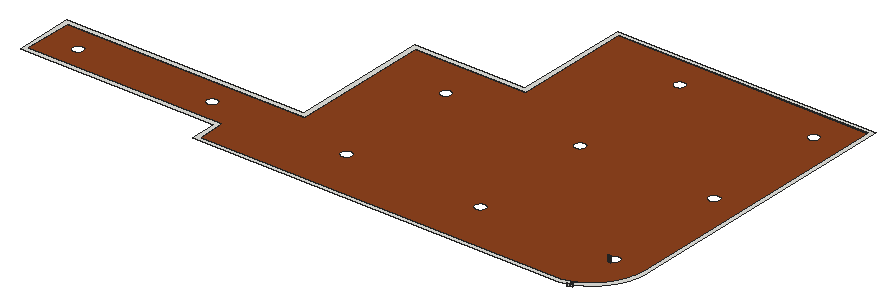
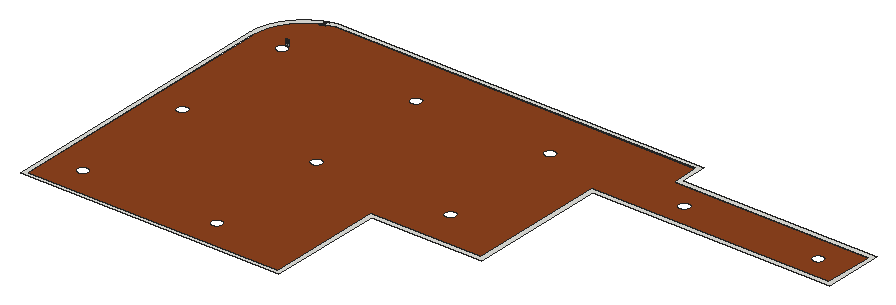
# SketchUp Ruby script. Lengths in inches.
U = 1.inch
M = Sketchup.active_model
def pt(a) = Geom::Point3d.new(a.map { |v| v * U })
def face(e, loops, mat)
  f = e.add_face(loops[0].map { |a| pt(a) })
  loops[1..].each { |l| e.add_face(l.map { |a| pt(a) }).erase! }
  f.material = f.back_material = mat if mat
  f
end
# faces: each face lists its corners as indices into pts; further lists are holes
def faces(e, pts, list, mat = nil) = list.each { |f| face(e, (f[0].is_a?(Array) ? f : [f]).map { |l| l.map { |i| pts[i] } }, mat) }
# xy, xz, yz: faces in a plane at the given z, y or x. An outline is a flat list of corners, or four numbers for a rectangle; further outlines are holes
def ring(l) = l.size == 4 ? [[l[0], l[1]], [l[2], l[1]], [l[2], l[3]], [l[0], l[3]]] : l.each_slice(2).to_a
def flat(e, list, mat, &to3) = list.each { |f| face(e, (f[0].is_a?(Array) ? f : [f]).map { |l| ring(l).map { |u, v| to3.(u, v) } }, mat) }
def xy(e, z, list, mat = nil) = flat(e, list, mat) { |x, y| [x, y, z] }
def xz(e, y, list, mat = nil) = flat(e, list, mat) { |x, z| [x, y, z] }
def yz(e, x, list, mat = nil) = flat(e, list, mat) { |y, z| [x, y, z] }
def lines(e, pts, list) = list.each { |a, b| e.add_line(pt(pts[a]), pt(pts[b])) }
# prism: a flat outline (further loops are holes) pulled along v
def prism(e, loops, v, mat = nil)
  f = face(e, loops, mat); d = Geom::Vector3d.new(v.map { |x| x * U })
  f.pushpull(f.normal.samedirection?(d) ? d.length : -d.length)
end
def box(e, o, s, mat = nil) = prism(e, [[o, [o[0] + s[0], o[1], o[2]], [o[0] + s[0], o[1] + s[1], o[2]], [o[0], o[1] + s[1], o[2]]]], [0, 0, s[2]], mat)
def at(x, y, z, deg = 0) = Geom::Transformation.translation(pt([x, y, z])) * Geom::Transformation.rotation(ORIGIN, Z_AXIS, deg.degrees)
def axes(o, x, y, z) = Geom::Transformation.new([*x, 0, *y, 0, *z, 0, *pt(o).to_a, 1])
def part(name) = M.definitions.add(name)
# library, detail: a bought-in or finely detailed component or shape, given as its bounding box
def library(name, o, s) = part(name).tap { |d| box(d.entities, o, s) }
def detail(e, o, s) = box(e.add_group.entities, o, s)
def put(e, d, t, mat = nil) = e.add_instance(d, t).tap { |i| i.material = mat if mat }
def group(e, t, mat = nil) = e.add_group.tap { |g| g.transformation = t; g.material = mat if mat }.entities
root = M.entities
M.materials.add("[Wood Fence]").color = [142, 67, 30]
xy(root,108,[[[135.5,161,135.5,175,35,175,35,201,158,201,158,273,215,273,215,333,345,333,345,186.92,344.99,186.68,344.98,186.4375,344.97,186.2,344.95,185.72,344.93,185.48,344.91,185.25,344.87,184.77,344.84,184.53,344.8125,184.29,344.78,184.06,344.72,183.58,344.68,183.35,344.64,183.11,344.6,182.875,344.5625,182.64,344.52,182.4,344.47,182.17,344.42,181.93,344.375,181.7,344.32,181.47,344.27,181.23,344.03,180.31,343.96,180.08,343.9,179.85,343.76,179.39,343.68,179.16,343.61,178.9375,343.53,178.71,343.45,178.48,343.375,178.26,343.29,178.03,343.21,177.81,343.03,177.37,342.94,177.14,342.85,176.92,342.75,176.7,342.66,176.48,342.56,176.27,342.46,176.05,342.35,175.83,342.25,175.62,342.14,175.4,342.04,175.19,341.93,174.98,341.8125,174.77,341.7,174.56,341.58,174.35,341.47,174.14,341.23,173.72,341.1,173.52,340.98,173.32,340.85,173.11,340.46,172.51,340.33,172.3125,340.19,172.12,340.06,171.92,339.92,171.72,339.78,171.53,339.63,171.34,339.49,171.15,339.34,170.96,339.2,170.77,339.05,170.58,338.9,170.4,338.75,170.21,338.59,170.03,338.4375,169.85,338.28,169.67,338.12,169.49,337.96,169.3125,337.8,169.13,337.63,168.96,337.47,168.79,337.3,168.62,337.13,168.44,336.97,168.28,336.79,168.11,336.62,167.94,336.45,167.78,336.27,167.62,336.1,167.46,335.56,166.98,335.375,166.83,335.19,166.67,335.01,166.52,334.63,166.22,334.44,166.08,334.25,165.93,333.87,165.65,333.67,165.51,333.48,165.37,333.28,165.23,332.08,164.45,331.87,164.33,331.67,164.21,331.04,163.85,330.83,163.74,330.62,163.625,330.41,163.52,330.2,163.41,329.98,163.3,329.77,163.19,329.55,163.09,329.34,162.99,328.9,162.79,328.68,162.7,328.46,162.6,328.02,162.42,327.79,162.34,327.57,162.25,327.35,162.17,327.12,162.08,326.9,162,326.67,161.93,326.44,161.85,326.22,161.78,325.99,161.7,325.76,161.64,325.3,161.5,324.84,161.375,324.61,161.32,324.14,161.2,323.68,161.1,323.44,161.05,323.21,161],[120.34,185,120.66,185,120.74,185.01,120.8125,185.02,120.89,185.03,121.05,185.05,121.125,185.07,121.2,185.08,121.28,185.1,121.35,185.125,121.43,185.15,121.5,185.17,121.58,185.2,121.79,185.29,121.86,185.33,121.93,185.36,122.07,185.44,122.13,185.48,122.2,185.53,122.26,185.57,122.33,185.62,122.57,185.82,122.62,185.88,122.68,185.93,122.88,186.17,122.93,186.24,122.97,186.3,123.02,186.37,123.06,186.43,123.14,186.57,123.17,186.64,123.21,186.71,123.3,186.92,123.33,187,123.35,187.07,123.375,187.15,123.4,187.22,123.42,187.3,123.43,187.375,123.45,187.45,123.47,187.61,123.48,187.6875,123.49,187.76,123.5,187.84,123.5,188.16,123.49,188.24,123.48,188.3125,123.47,188.39,123.45,188.55,123.43,188.625,123.42,188.7,123.4,188.78,123.375,188.85,123.35,188.93,123.33,189,123.3,189.08,123.21,189.29,123.17,189.36,123.14,189.43,123.06,189.57,123.02,189.63,122.97,189.7,122.93,189.76,122.88,189.83,122.68,190.07,122.62,190.12,122.57,190.18,122.33,190.38,122.26,190.43,122.2,190.47,122.13,190.52,122.07,190.56,121.93,190.64,121.86,190.67,121.79,190.71,121.58,190.8,121.5,190.83,121.43,190.85,121.35,190.875,121.28,190.9,121.2,190.92,121.125,190.93,121.05,190.95,120.89,190.97,120.8125,190.98,120.74,190.99,120.66,191,120.34,191,120.26,190.99,120.1875,190.98,120.11,190.97,119.95,190.95,119.875,190.93,119.8,190.92,119.72,190.9,119.65,190.875,119.57,190.85,119.5,190.83,119.42,190.8,119.21,190.71,119.14,190.67,119.07,190.64,118.93,190.56,118.87,190.52,118.8,190.47,118.74,190.43,118.67,190.38,118.43,190.18,118.38,190.12,118.32,190.07,118.12,189.83,118.07,189.76,118.03,189.7,117.98,189.63,117.94,189.57,117.86,189.43,117.83,189.36,117.79,189.29,117.7,189.08,117.67,189,117.65,188.93,117.625,188.85,117.6,188.78,117.58,188.7,117.57,188.625,117.55,188.55,117.53,188.39,117.52,188.3125,117.51,188.24,117.5,188.16,117.5,187.84,117.51,187.76,117.52,187.6875,117.53,187.61,117.55,187.45,117.57,187.375,117.58,187.3,117.6,187.22,117.625,187.15,117.65,187.07,117.67,187,117.7,186.92,117.79,186.71,117.83,186.64,117.86,186.57,117.94,186.43,117.98,186.37,118.03,186.3,118.07,186.24,118.12,186.17,118.32,185.93,118.38,185.88,118.43,185.82,118.67,185.62,118.74,185.57,118.8,185.53,118.87,185.48,118.93,185.44,119.07,185.36,119.14,185.33,119.21,185.29,119.42,185.2,119.5,185.17,119.57,185.15,119.65,185.125,119.72,185.1,119.8,185.08,119.875,185.07,119.95,185.05,120.11,185.03,120.1875,185.02,120.26,185.01],[259.34,314,259.66,314,259.74,314.01,259.8125,314.02,259.89,314.03,260.05,314.05,260.125,314.07,260.2,314.08,260.28,314.1,260.35,314.125,260.43,314.15,260.5,314.17,260.58,314.2,260.79,314.29,260.86,314.33,260.93,314.36,261.07,314.44,261.13,314.48,261.2,314.53,261.26,314.57,261.33,314.62,261.57,314.82,261.62,314.88,261.68,314.93,261.88,315.17,261.93,315.24,261.97,315.3,262.02,315.37,262.06,315.43,262.14,315.57,262.17,315.64,262.21,315.71,262.3,315.92,262.33,316,262.35,316.07,262.375,316.15,262.4,316.22,262.42,316.3,262.43,316.375,262.45,316.45,262.47,316.61,262.48,316.6875,262.49,316.76,262.5,316.84,262.5,317.16,262.49,317.24,262.48,317.3125,262.47,317.39,262.45,317.55,262.43,317.625,262.42,317.7,262.4,317.78,262.375,317.85,262.35,317.93,262.33,318,262.3,318.08,262.21,318.29,262.17,318.36,262.14,318.43,262.06,318.57,262.02,318.63,261.97,318.7,261.93,318.76,261.88,318.83,261.68,319.07,261.62,319.12,261.57,319.18,261.33,319.38,261.26,319.43,261.2,319.47,261.13,319.52,261.07,319.56,260.93,319.64,260.86,319.67,260.79,319.71,260.58,319.8,260.5,319.83,260.43,319.85,260.35,319.875,260.28,319.9,260.2,319.92,260.125,319.93,260.05,319.95,259.89,319.97,259.8125,319.98,259.74,319.99,259.66,320,259.34,320,259.26,319.99,259.1875,319.98,259.11,319.97,258.95,319.95,258.875,319.93,258.8,319.92,258.72,319.9,258.65,319.875,258.57,319.85,258.5,319.83,258.42,319.8,258.21,319.71,258.14,319.67,258.07,319.64,257.93,319.56,257.87,319.52,257.8,319.47,257.74,319.43,257.67,319.38,257.43,319.18,257.38,319.12,257.32,319.07,257.12,318.83,257.07,318.76,257.03,318.7,256.98,318.63,256.94,318.57,256.86,318.43,256.83,318.36,256.79,318.29,256.7,318.08,256.67,318,256.65,317.93,256.625,317.85,256.6,317.78,256.58,317.7,256.57,317.625,256.55,317.55,256.53,317.39,256.52,317.3125,256.51,317.24,256.5,317.16,256.5,316.84,256.51,316.76,256.52,316.6875,256.53,316.61,256.55,316.45,256.57,316.375,256.58,316.3,256.6,316.22,256.625,316.15,256.65,316.07,256.67,316,256.7,315.92,256.79,315.71,256.83,315.64,256.86,315.57,256.94,315.43,256.98,315.37,257.03,315.3,257.07,315.24,257.12,315.17,257.32,314.93,257.38,314.88,257.43,314.82,257.67,314.62,257.74,314.57,257.8,314.53,257.87,314.48,257.93,314.44,258.07,314.36,258.14,314.33,258.21,314.29,258.42,314.2,258.5,314.17,258.57,314.15,258.65,314.125,258.72,314.1,258.8,314.08,258.875,314.07,258.95,314.05,259.11,314.03,259.1875,314.02,259.26,314.01],[328.84,314,329.16,314,329.24,314.01,329.3125,314.02,329.39,314.03,329.55,314.05,329.625,314.07,329.7,314.08,329.78,314.1,329.85,314.125,329.93,314.15,330,314.17,330.08,314.2,330.29,314.29,330.36,314.33,330.43,314.36,330.57,314.44,330.63,314.48,330.7,314.53,330.76,314.57,330.83,314.62,331.07,314.82,331.12,314.88,331.18,314.93,331.38,315.17,331.43,315.24,331.47,315.3,331.52,315.37,331.56,315.43,331.64,315.57,331.67,315.64,331.71,315.71,331.8,315.92,331.83,316,331.85,316.07,331.875,316.15,331.9,316.22,331.92,316.3,331.93,316.375,331.95,316.45,331.97,316.61,331.98,316.6875,331.99,316.76,332,316.84,332,317.16,331.99,317.24,331.98,317.3125,331.97,317.39,331.95,317.55,331.93,317.625,331.92,317.7,331.9,317.78,331.875,317.85,331.85,317.93,331.83,318,331.8,318.08,331.71,318.29,331.67,318.36,331.64,318.43,331.56,318.57,331.52,318.63,331.47,318.7,331.43,318.76,331.38,318.83,331.18,319.07,331.12,319.12,331.07,319.18,330.83,319.38,330.76,319.43,330.7,319.47,330.63,319.52,330.57,319.56,330.43,319.64,330.36,319.67,330.29,319.71,330.08,319.8,330,319.83,329.93,319.85,329.85,319.875,329.78,319.9,329.7,319.92,329.625,319.93,329.55,319.95,329.39,319.97,329.3125,319.98,329.24,319.99,329.16,320,328.84,320,328.76,319.99,328.6875,319.98,328.61,319.97,328.45,319.95,328.375,319.93,328.3,319.92,328.22,319.9,328.15,319.875,328.07,319.85,328,319.83,327.92,319.8,327.71,319.71,327.64,319.67,327.57,319.64,327.43,319.56,327.37,319.52,327.3,319.47,327.24,319.43,327.17,319.38,326.93,319.18,326.88,319.12,326.82,319.07,326.62,318.83,326.57,318.76,326.53,318.7,326.48,318.63,326.44,318.57,326.36,318.43,326.33,318.36,326.29,318.29,326.2,318.08,326.17,318,326.15,317.93,326.125,317.85,326.1,317.78,326.08,317.7,326.07,317.625,326.05,317.55,326.03,317.39,326.02,317.3125,326.01,317.24,326,317.16,326,316.84,326.01,316.76,326.02,316.6875,326.03,316.61,326.05,316.45,326.07,316.375,326.08,316.3,326.1,316.22,326.125,316.15,326.15,316.07,326.17,316,326.2,315.92,326.29,315.71,326.33,315.64,326.36,315.57,326.44,315.43,326.48,315.37,326.53,315.3,326.57,315.24,326.62,315.17,326.82,314.93,326.88,314.88,326.93,314.82,327.17,314.62,327.24,314.57,327.3,314.53,327.37,314.48,327.43,314.44,327.57,314.36,327.64,314.33,327.71,314.29,327.92,314.2,328,314.17,328.07,314.15,328.15,314.125,328.22,314.1,328.3,314.08,328.375,314.07,328.45,314.05,328.61,314.03,328.6875,314.02,328.76,314.01],[259.34,249.5,259.66,249.5,259.74,249.51,259.8125,249.52,259.89,249.53,260.05,249.55,260.125,249.57,260.2,249.58,260.28,249.6,260.35,249.625,260.43,249.65,260.5,249.67,260.58,249.7,260.79,249.79,260.86,249.83,260.93,249.86,261.07,249.94,261.13,249.98,261.2,250.03,261.26,250.07,261.33,250.12,261.57,250.32,261.62,250.38,261.68,250.43,261.88,250.67,261.93,250.74,261.97,250.8,262.02,250.87,262.06,250.93,262.14,251.07,262.17,251.14,262.21,251.21,262.3,251.42,262.33,251.5,262.35,251.57,262.375,251.65,262.4,251.72,262.42,251.8,262.43,251.875,262.45,251.95,262.47,252.11,262.48,252.1875,262.49,252.26,262.5,252.34,262.5,252.66,262.49,252.74,262.48,252.8125,262.47,252.89,262.45,253.05,262.43,253.125,262.42,253.2,262.4,253.28,262.375,253.35,262.35,253.43,262.33,253.5,262.3,253.58,262.21,253.79,262.17,253.86,262.14,253.93,262.06,254.07,262.02,254.13,261.97,254.2,261.93,254.26,261.88,254.33,261.68,254.57,261.62,254.62,261.57,254.68,261.33,254.88,261.26,254.93,261.2,254.97,261.13,255.02,261.07,255.06,260.93,255.14,260.86,255.17,260.79,255.21,260.58,255.3,260.5,255.33,260.43,255.35,260.35,255.375,260.28,255.4,260.2,255.42,260.125,255.43,260.05,255.45,259.89,255.47,259.8125,255.48,259.74,255.49,259.66,255.5,259.34,255.5,259.26,255.49,259.1875,255.48,259.11,255.47,258.95,255.45,258.875,255.43,258.8,255.42,258.72,255.4,258.65,255.375,258.57,255.35,258.5,255.33,258.42,255.3,258.21,255.21,258.14,255.17,258.07,255.14,257.93,255.06,257.87,255.02,257.8,254.97,257.74,254.93,257.67,254.88,257.43,254.68,257.38,254.62,257.32,254.57,257.12,254.33,257.07,254.26,257.03,254.2,256.98,254.13,256.94,254.07,256.86,253.93,256.83,253.86,256.79,253.79,256.7,253.58,256.67,253.5,256.65,253.43,256.625,253.35,256.6,253.28,256.58,253.2,256.57,253.125,256.55,253.05,256.53,252.89,256.52,252.8125,256.51,252.74,256.5,252.66,256.5,252.34,256.51,252.26,256.52,252.1875,256.53,252.11,256.55,251.95,256.57,251.875,256.58,251.8,256.6,251.72,256.625,251.65,256.65,251.57,256.67,251.5,256.7,251.42,256.79,251.21,256.83,251.14,256.86,251.07,256.94,250.93,256.98,250.87,257.03,250.8,257.07,250.74,257.12,250.67,257.32,250.43,257.38,250.38,257.43,250.32,257.67,250.12,257.74,250.07,257.8,250.03,257.87,249.98,257.93,249.94,258.07,249.86,258.14,249.83,258.21,249.79,258.42,249.7,258.5,249.67,258.57,249.65,258.65,249.625,258.72,249.6,258.8,249.58,258.875,249.57,258.95,249.55,259.11,249.53,259.1875,249.52,259.26,249.51],[328.84,249.5,329.16,249.5,329.24,249.51,329.3125,249.52,329.39,249.53,329.55,249.55,329.625,249.57,329.7,249.58,329.78,249.6,329.85,249.625,329.93,249.65,330,249.67,330.08,249.7,330.29,249.79,330.36,249.83,330.43,249.86,330.57,249.94,330.63,249.98,330.7,250.03,330.76,250.07,330.83,250.12,331.07,250.32,331.12,250.38,331.18,250.43,331.38,250.67,331.43,250.74,331.47,250.8,331.52,250.87,331.56,250.93,331.64,251.07,331.67,251.14,331.71,251.21,331.8,251.42,331.83,251.5,331.85,251.57,331.875,251.65,331.9,251.72,331.92,251.8,331.93,251.875,331.95,251.95,331.97,252.11,331.98,252.1875,331.99,252.26,332,252.34,332,252.66,331.99,252.74,331.98,252.8125,331.97,252.89,331.95,253.05,331.93,253.125,331.92,253.2,331.9,253.28,331.875,253.35,331.85,253.43,331.83,253.5,331.8,253.58,331.71,253.79,331.67,253.86,331.64,253.93,331.56,254.07,331.52,254.13,331.47,254.2,331.43,254.26,331.38,254.33,331.18,254.57,331.12,254.62,331.07,254.68,330.83,254.88,330.76,254.93,330.7,254.97,330.63,255.02,330.57,255.06,330.43,255.14,330.36,255.17,330.29,255.21,330.08,255.3,330,255.33,329.93,255.35,329.85,255.375,329.78,255.4,329.7,255.42,329.625,255.43,329.55,255.45,329.39,255.47,329.3125,255.48,329.24,255.49,329.16,255.5,328.84,255.5,328.76,255.49,328.6875,255.48,328.61,255.47,328.45,255.45,328.375,255.43,328.3,255.42,328.22,255.4,328.15,255.375,328.07,255.35,328,255.33,327.92,255.3,327.71,255.21,327.64,255.17,327.57,255.14,327.43,255.06,327.37,255.02,327.3,254.97,327.24,254.93,327.17,254.88,326.93,254.68,326.88,254.62,326.82,254.57,326.62,254.33,326.57,254.26,326.53,254.2,326.48,254.13,326.44,254.07,326.36,253.93,326.33,253.86,326.29,253.79,326.2,253.58,326.17,253.5,326.15,253.43,326.125,253.35,326.1,253.28,326.08,253.2,326.07,253.125,326.05,253.05,326.03,252.89,326.02,252.8125,326.01,252.74,326,252.66,326,252.34,326.01,252.26,326.02,252.1875,326.03,252.11,326.05,251.95,326.07,251.875,326.08,251.8,326.1,251.72,326.125,251.65,326.15,251.57,326.17,251.5,326.2,251.42,326.29,251.21,326.33,251.14,326.36,251.07,326.44,250.93,326.48,250.87,326.53,250.8,326.57,250.74,326.62,250.67,326.82,250.43,326.88,250.38,326.93,250.32,327.17,250.12,327.24,250.07,327.3,250.03,327.37,249.98,327.43,249.94,327.57,249.86,327.64,249.83,327.71,249.79,327.92,249.7,328,249.67,328.07,249.65,328.15,249.625,328.22,249.6,328.3,249.58,328.375,249.57,328.45,249.55,328.61,249.53,328.6875,249.52,328.76,249.51],[259.34,185,259.66,185,259.74,185.01,259.8125,185.02,259.89,185.03,260.05,185.05,260.125,185.07,260.2,185.08,260.28,185.1,260.35,185.125,260.43,185.15,260.5,185.17,260.58,185.2,260.79,185.29,260.86,185.33,260.93,185.36,261.07,185.44,261.13,185.48,261.2,185.53,261.26,185.57,261.33,185.62,261.57,185.82,261.62,185.88,261.68,185.93,261.88,186.17,261.93,186.24,261.97,186.3,262.02,186.37,262.06,186.43,262.14,186.57,262.17,186.64,262.21,186.71,262.3,186.92,262.33,187,262.35,187.07,262.375,187.15,262.4,187.22,262.42,187.3,262.43,187.375,262.45,187.45,262.47,187.61,262.48,187.6875,262.49,187.76,262.5,187.84,262.5,188.16,262.49,188.24,262.48,188.3125,262.47,188.39,262.45,188.55,262.43,188.625,262.42,188.7,262.4,188.78,262.375,188.85,262.35,188.93,262.33,189,262.3,189.08,262.21,189.29,262.17,189.36,262.14,189.43,262.06,189.57,262.02,189.63,261.97,189.7,261.93,189.76,261.88,189.83,261.68,190.07,261.62,190.12,261.57,190.18,261.33,190.38,261.26,190.43,261.2,190.47,261.13,190.52,261.07,190.56,260.93,190.64,260.86,190.67,260.79,190.71,260.58,190.8,260.5,190.83,260.43,190.85,260.35,190.875,260.28,190.9,260.2,190.92,260.125,190.93,260.05,190.95,259.89,190.97,259.8125,190.98,259.74,190.99,259.66,191,259.34,191,259.26,190.99,259.1875,190.98,259.11,190.97,258.95,190.95,258.875,190.93,258.8,190.92,258.72,190.9,258.65,190.875,258.57,190.85,258.5,190.83,258.42,190.8,258.21,190.71,258.14,190.67,258.07,190.64,257.93,190.56,257.87,190.52,257.8,190.47,257.74,190.43,257.67,190.38,257.43,190.18,257.38,190.12,257.32,190.07,257.12,189.83,257.07,189.76,257.03,189.7,256.98,189.63,256.94,189.57,256.86,189.43,256.83,189.36,256.79,189.29,256.7,189.08,256.67,189,256.65,188.93,256.625,188.85,256.6,188.78,256.58,188.7,256.57,188.625,256.55,188.55,256.53,188.39,256.52,188.3125,256.51,188.24,256.5,188.16,256.5,187.84,256.51,187.76,256.52,187.6875,256.53,187.61,256.55,187.45,256.57,187.375,256.58,187.3,256.6,187.22,256.625,187.15,256.65,187.07,256.67,187,256.7,186.92,256.79,186.71,256.83,186.64,256.86,186.57,256.94,186.43,256.98,186.37,257.03,186.3,257.07,186.24,257.12,186.17,257.32,185.93,257.38,185.88,257.43,185.82,257.67,185.62,257.74,185.57,257.8,185.53,257.87,185.48,257.93,185.44,258.07,185.36,258.14,185.33,258.21,185.29,258.42,185.2,258.5,185.17,258.57,185.15,258.65,185.125,258.72,185.1,258.8,185.08,258.875,185.07,258.95,185.05,259.11,185.03,259.1875,185.02,259.26,185.01],[328.84,185,329.16,185,329.24,185.01,329.3125,185.02,329.39,185.03,329.55,185.05,329.625,185.07,329.7,185.08,329.78,185.1,329.85,185.125,329.93,185.15,330,185.17,330.08,185.2,330.29,185.29,330.36,185.33,330.43,185.36,330.57,185.44,330.63,185.48,330.7,185.53,330.76,185.57,330.83,185.62,331.07,185.82,331.12,185.88,331.18,185.93,331.38,186.17,331.43,186.24,331.47,186.3,331.52,186.37,331.56,186.43,331.64,186.57,331.67,186.64,331.71,186.71,331.8,186.92,331.83,187,331.85,187.07,331.875,187.15,331.9,187.22,331.92,187.3,331.93,187.375,331.95,187.45,331.97,187.61,331.98,187.6875,331.99,187.76,332,187.84,332,188.16,331.99,188.24,331.98,188.3125,331.97,188.39,331.95,188.55,331.93,188.625,331.92,188.7,331.9,188.78,331.875,188.85,331.85,188.93,331.83,189,331.8,189.08,331.71,189.29,331.67,189.36,331.64,189.43,331.56,189.57,331.52,189.63,331.47,189.7,331.43,189.76,331.38,189.83,331.18,190.07,331.12,190.12,331.07,190.18,330.83,190.38,330.76,190.43,330.7,190.47,330.63,190.52,330.57,190.56,330.43,190.64,330.36,190.67,330.29,190.71,330.08,190.8,330,190.83,329.93,190.85,329.85,190.875,329.78,190.9,329.7,190.92,329.625,190.93,329.55,190.95,329.39,190.97,329.3125,190.98,329.24,190.99,329.16,191,328.84,191,328.76,190.99,328.6875,190.98,328.61,190.97,328.45,190.95,328.375,190.93,328.3,190.92,328.22,190.9,328.15,190.875,328.07,190.85,328,190.83,327.92,190.8,327.71,190.71,327.64,190.67,327.57,190.64,327.43,190.56,327.37,190.52,327.3,190.47,327.24,190.43,327.17,190.38,326.93,190.18,326.88,190.12,326.82,190.07,326.62,189.83,326.57,189.76,326.53,189.7,326.48,189.63,326.44,189.57,326.36,189.43,326.33,189.36,326.29,189.29,326.2,189.08,326.17,189,326.15,188.93,326.125,188.85,326.1,188.78,326.08,188.7,326.07,188.625,326.05,188.55,326.03,188.39,326.02,188.3125,326.01,188.24,326,188.16,326,187.84,326.01,187.76,326.02,187.6875,326.03,187.61,326.05,187.45,326.07,187.375,326.08,187.3,326.1,187.22,326.125,187.15,326.15,187.07,326.17,187,326.2,186.92,326.29,186.71,326.33,186.64,326.36,186.57,326.44,186.43,326.48,186.37,326.53,186.3,326.57,186.24,326.62,186.17,326.82,185.93,326.88,185.88,326.93,185.82,327.17,185.62,327.24,185.57,327.3,185.53,327.37,185.48,327.43,185.44,327.57,185.36,327.64,185.33,327.71,185.29,327.92,185.2,328,185.17,328.07,185.15,328.15,185.125,328.22,185.1,328.3,185.08,328.375,185.07,328.45,185.05,328.61,185.03,328.6875,185.02,328.76,185.01],[50.84,185,51.16,185,51.24,185.01,51.3125,185.02,51.39,185.03,51.55,185.05,51.625,185.07,51.7,185.08,51.78,185.1,51.85,185.125,51.93,185.15,52,185.17,52.08,185.2,52.29,185.29,52.36,185.33,52.43,185.36,52.57,185.44,52.63,185.48,52.7,185.53,52.76,185.57,52.83,185.62,53.07,185.82,53.12,185.88,53.18,185.93,53.38,186.17,53.43,186.24,53.47,186.3,53.52,186.37,53.56,186.43,53.64,186.57,53.67,186.64,53.71,186.71,53.8,186.92,53.83,187,53.85,187.07,53.875,187.15,53.9,187.22,53.92,187.3,53.93,187.375,53.95,187.45,53.97,187.61,53.98,187.6875,53.99,187.76,54,187.84,54,188.16,53.99,188.24,53.98,188.3125,53.97,188.39,53.95,188.55,53.93,188.625,53.92,188.7,53.9,188.78,53.875,188.85,53.85,188.93,53.83,189,53.8,189.08,53.71,189.29,53.67,189.36,53.64,189.43,53.56,189.57,53.52,189.63,53.47,189.7,53.43,189.76,53.38,189.83,53.18,190.07,53.12,190.12,53.07,190.18,52.83,190.38,52.76,190.43,52.7,190.47,52.63,190.52,52.57,190.56,52.43,190.64,52.36,190.67,52.29,190.71,52.08,190.8,52,190.83,51.93,190.85,51.85,190.875,51.78,190.9,51.7,190.92,51.625,190.93,51.55,190.95,51.39,190.97,51.3125,190.98,51.24,190.99,51.16,191,50.84,191,50.76,190.99,50.6875,190.98,50.61,190.97,50.45,190.95,50.375,190.93,50.3,190.92,50.22,190.9,50.15,190.875,50.07,190.85,50,190.83,49.92,190.8,49.71,190.71,49.64,190.67,49.57,190.64,49.43,190.56,49.37,190.52,49.3,190.47,49.24,190.43,49.17,190.38,48.93,190.18,48.88,190.12,48.82,190.07,48.62,189.83,48.57,189.76,48.53,189.7,48.48,189.63,48.44,189.57,48.36,189.43,48.33,189.36,48.29,189.29,48.2,189.08,48.17,189,48.15,188.93,48.125,188.85,48.1,188.78,48.08,188.7,48.07,188.625,48.05,188.55,48.03,188.39,48.02,188.3125,48.01,188.24,48,188.16,48,187.84,48.01,187.76,48.02,187.6875,48.03,187.61,48.05,187.45,48.07,187.375,48.08,187.3,48.1,187.22,48.125,187.15,48.15,187.07,48.17,187,48.2,186.92,48.29,186.71,48.33,186.64,48.36,186.57,48.44,186.43,48.48,186.37,48.53,186.3,48.57,186.24,48.62,186.17,48.82,185.93,48.88,185.88,48.93,185.82,49.17,185.62,49.24,185.57,49.3,185.53,49.37,185.48,49.43,185.44,49.57,185.36,49.64,185.33,49.71,185.29,49.92,185.2,50,185.17,50.07,185.15,50.15,185.125,50.22,185.1,50.3,185.08,50.375,185.07,50.45,185.05,50.61,185.03,50.6875,185.02,50.76,185.01],[189.84,185,190.16,185,190.24,185.01,190.3125,185.02,190.39,185.03,190.55,185.05,190.625,185.07,190.7,185.08,190.78,185.1,190.85,185.125,190.93,185.15,191,185.17,191.08,185.2,191.29,185.29,191.36,185.33,191.43,185.36,191.57,185.44,191.63,185.48,191.7,185.53,191.76,185.57,191.83,185.62,192.07,185.82,192.12,185.88,192.18,185.93,192.38,186.17,192.43,186.24,192.47,186.3,192.52,186.37,192.56,186.43,192.64,186.57,192.67,186.64,192.71,186.71,192.8,186.92,192.83,187,192.85,187.07,192.875,187.15,192.9,187.22,192.92,187.3,192.93,187.375,192.95,187.45,192.97,187.61,192.98,187.6875,192.99,187.76,193,187.84,193,188.16,192.99,188.24,192.98,188.3125,192.97,188.39,192.95,188.55,192.93,188.625,192.92,188.7,192.9,188.78,192.875,188.85,192.85,188.93,192.83,189,192.8,189.08,192.71,189.29,192.67,189.36,192.64,189.43,192.56,189.57,192.52,189.63,192.47,189.7,192.43,189.76,192.38,189.83,192.18,190.07,192.12,190.12,192.07,190.18,191.83,190.38,191.76,190.43,191.7,190.47,191.63,190.52,191.57,190.56,191.43,190.64,191.36,190.67,191.29,190.71,191.08,190.8,191,190.83,190.93,190.85,190.85,190.875,190.78,190.9,190.7,190.92,190.625,190.93,190.55,190.95,190.39,190.97,190.3125,190.98,190.24,190.99,190.16,191,189.84,191,189.76,190.99,189.6875,190.98,189.61,190.97,189.45,190.95,189.375,190.93,189.3,190.92,189.22,190.9,189.15,190.875,189.07,190.85,189,190.83,188.92,190.8,188.71,190.71,188.64,190.67,188.57,190.64,188.43,190.56,188.37,190.52,188.3,190.47,188.24,190.43,188.17,190.38,187.93,190.18,187.88,190.12,187.82,190.07,187.62,189.83,187.57,189.76,187.53,189.7,187.48,189.63,187.44,189.57,187.36,189.43,187.33,189.36,187.29,189.29,187.2,189.08,187.17,189,187.15,188.93,187.125,188.85,187.1,188.78,187.08,188.7,187.07,188.625,187.05,188.55,187.03,188.39,187.02,188.3125,187.01,188.24,187,188.16,187,187.84,187.01,187.76,187.02,187.6875,187.03,187.61,187.05,187.45,187.07,187.375,187.08,187.3,187.1,187.22,187.125,187.15,187.15,187.07,187.17,187,187.2,186.92,187.29,186.71,187.33,186.64,187.36,186.57,187.44,186.43,187.48,186.37,187.53,186.3,187.57,186.24,187.62,186.17,187.82,185.93,187.88,185.88,187.93,185.82,188.17,185.62,188.24,185.57,188.3,185.53,188.37,185.48,188.43,185.44,188.57,185.36,188.64,185.33,188.71,185.29,188.92,185.2,189,185.17,189.07,185.15,189.15,185.125,189.22,185.1,189.3,185.08,189.375,185.07,189.45,185.05,189.61,185.03,189.6875,185.02,189.76,185.01],[189.84,249.5,190.16,249.5,190.24,249.51,190.3125,249.52,190.39,249.53,190.55,249.55,190.625,249.57,190.7,249.58,190.78,249.6,190.85,249.625,190.93,249.65,191,249.67,191.08,249.7,191.29,249.79,191.36,249.83,191.43,249.86,191.57,249.94,191.63,249.98,191.7,250.03,191.76,250.07,191.83,250.12,192.07,250.32,192.12,250.38,192.18,250.43,192.38,250.67,192.43,250.74,192.47,250.8,192.52,250.87,192.56,250.93,192.64,251.07,192.67,251.14,192.71,251.21,192.8,251.42,192.83,251.5,192.85,251.57,192.875,251.65,192.9,251.72,192.92,251.8,192.93,251.875,192.95,251.95,192.97,252.11,192.98,252.1875,192.99,252.26,193,252.34,193,252.66,192.99,252.74,192.98,252.8125,192.97,252.89,192.95,253.05,192.93,253.125,192.92,253.2,192.9,253.28,192.875,253.35,192.85,253.43,192.83,253.5,192.8,253.58,192.71,253.79,192.67,253.86,192.64,253.93,192.56,254.07,192.52,254.13,192.47,254.2,192.43,254.26,192.38,254.33,192.18,254.57,192.12,254.62,192.07,254.68,191.83,254.88,191.76,254.93,191.7,254.97,191.63,255.02,191.57,255.06,191.43,255.14,191.36,255.17,191.29,255.21,191.08,255.3,191,255.33,190.93,255.35,190.85,255.375,190.78,255.4,190.7,255.42,190.625,255.43,190.55,255.45,190.39,255.47,190.3125,255.48,190.24,255.49,190.16,255.5,189.84,255.5,189.76,255.49,189.6875,255.48,189.61,255.47,189.45,255.45,189.375,255.43,189.3,255.42,189.22,255.4,189.15,255.375,189.07,255.35,189,255.33,188.92,255.3,188.71,255.21,188.64,255.17,188.57,255.14,188.43,255.06,188.37,255.02,188.3,254.97,188.24,254.93,188.17,254.88,187.93,254.68,187.88,254.62,187.82,254.57,187.62,254.33,187.57,254.26,187.53,254.2,187.48,254.13,187.44,254.07,187.36,253.93,187.33,253.86,187.29,253.79,187.2,253.58,187.17,253.5,187.15,253.43,187.125,253.35,187.1,253.28,187.08,253.2,187.07,253.125,187.05,253.05,187.03,252.89,187.02,252.8125,187.01,252.74,187,252.66,187,252.34,187.01,252.26,187.02,252.1875,187.03,252.11,187.05,251.95,187.07,251.875,187.08,251.8,187.1,251.72,187.125,251.65,187.15,251.57,187.17,251.5,187.2,251.42,187.29,251.21,187.33,251.14,187.36,251.07,187.44,250.93,187.48,250.87,187.53,250.8,187.57,250.74,187.62,250.67,187.82,250.43,187.88,250.38,187.93,250.32,188.17,250.12,188.24,250.07,188.3,250.03,188.37,249.98,188.43,249.94,188.57,249.86,188.64,249.83,188.71,249.79,188.92,249.7,189,249.67,189.07,249.65,189.15,249.625,189.22,249.6,189.3,249.58,189.375,249.57,189.45,249.55,189.61,249.53,189.6875,249.52,189.76,249.51]]],"[Wood Fence]")
xy(root,108.5,[[[133.5,159,133.5,173,33,173,33,203,156,203,156,275,213,275,213,335,347,335,347,186.875,346.99,186.62,346.97,186.1,346.96,185.85,346.94,185.59,346.92,185.34,346.88,184.82,346.86,184.57,346.83,184.3125,346.8,184.06,346.77,183.8,346.73,183.55,346.7,183.29,346.62,182.79,346.58,182.53,346.48,182.03,346.43,181.77,346.33,181.27,346.09,180.27,346.02,180.02,345.96,179.78,345.82,179.28,345.74,179.04,345.67,178.79,345.59,178.55,345.51,178.3,345.42,178.06,345.34,177.82,345.25,177.57,344.98,176.85,344.88,176.61,344.79,176.375,344.6875,176.14,344.59,175.9,344.48,175.67,344.375,175.43,344.27,175.2,344.05,174.74,343.93,174.51,343.82,174.28,343.58,173.82,343.46,173.6,343.33,173.37,343.21,173.15,343.08,172.93,342.95,172.7,342.82,172.48,342.68,172.27,342.55,172.05,342.27,171.61,342.125,171.4,341.98,171.1875,341.84,170.98,341.24,170.14,341.08,169.9375,340.93,169.73,340.45,169.13,340.28,168.93,340.12,168.74,339.95,168.54,339.78,168.35,339.61,168.15,339.4375,167.96,339.26,167.77,339.09,167.59,338.91,167.4,338.73,167.22,338.55,167.03,338.37,166.85,338.1875,166.67,338,166.49,337.8125,166.32,337.625,166.14,337.4375,165.97,337.24,165.8,336.86,165.46,336.66,165.3,336.46,165.13,336.26,164.97,336.0625,164.81,335.86,164.65,335.66,164.49,335.46,164.34,335.25,164.18,334.83,163.88,334.625,163.73,334.41,163.59,334.2,163.44,333.99,163.3,333.55,163.02,333.34,162.88,333.12,162.75,332.9,162.61,332.46,162.35,332.23,162.23,332.01,162.1,331.78,161.98,331.56,161.86,331.1,161.62,330.87,161.51,330.64,161.39,330.41,161.28,330.17,161.17,329.94,161.07,329.71,160.96,329.23,160.76,329,160.66,328.76,160.57,328.52,160.47,327.8,160.2,327.56,160.12,327.3125,160.03,327.07,159.95,326.83,159.87,326.58,159.79,326.33,159.72,326.09,159.65,325.34,159.44,325.1,159.38,324.1,159.14,323.84,159.09,323.59,159.04,323.38,159],[135.5,161,323.21,161,323.44,161.05,323.68,161.1,324.14,161.2,324.61,161.32,324.84,161.375,325.3,161.5,325.76,161.64,325.99,161.7,326.22,161.78,326.44,161.85,326.67,161.93,326.9,162,327.12,162.08,327.35,162.17,327.57,162.25,327.79,162.34,328.02,162.42,328.46,162.6,328.68,162.7,328.9,162.79,329.34,162.99,329.55,163.09,329.77,163.19,329.98,163.3,330.2,163.41,330.41,163.52,330.62,163.625,330.83,163.74,331.04,163.85,331.67,164.21,331.87,164.33,332.08,164.45,333.28,165.23,333.48,165.37,333.67,165.51,333.87,165.65,334.25,165.93,334.44,166.08,334.63,166.22,335.01,166.52,335.19,166.67,335.375,166.83,335.56,166.98,336.1,167.46,336.27,167.62,336.45,167.78,336.62,167.94,336.79,168.11,336.97,168.28,337.13,168.44,337.3,168.62,337.47,168.79,337.63,168.96,337.8,169.13,337.96,169.3125,338.12,169.49,338.28,169.67,338.4375,169.85,338.59,170.03,338.75,170.21,338.9,170.4,339.05,170.58,339.2,170.77,339.34,170.96,339.49,171.15,339.63,171.34,339.78,171.53,339.92,171.72,340.06,171.92,340.19,172.12,340.33,172.3125,340.46,172.51,340.85,173.11,340.98,173.32,341.1,173.52,341.23,173.72,341.47,174.14,341.58,174.35,341.7,174.56,341.8125,174.77,341.93,174.98,342.04,175.19,342.14,175.4,342.25,175.62,342.35,175.83,342.46,176.05,342.56,176.27,342.66,176.48,342.75,176.7,342.85,176.92,342.94,177.14,343.03,177.37,343.21,177.81,343.29,178.03,343.375,178.26,343.45,178.48,343.53,178.71,343.61,178.9375,343.68,179.16,343.76,179.39,343.9,179.85,343.96,180.08,344.03,180.31,344.27,181.23,344.32,181.47,344.375,181.7,344.42,181.93,344.47,182.17,344.52,182.4,344.5625,182.64,344.6,182.875,344.64,183.11,344.68,183.35,344.72,183.58,344.78,184.06,344.8125,184.29,344.84,184.53,344.87,184.77,344.91,185.25,344.93,185.48,344.95,185.72,344.97,186.2,344.98,186.4375,344.99,186.68,345,186.92,345,333,215,333,215,273,158,273,158,201,35,201,35,175,135.5,175]]])
xz(root,185,[[328.84,108,328.92,111],[328.92,108,329,111],[329,108,329.08,111],[329.08,108,329.16,111]])
p = [[327.07,159.95,107.5],[326.83,159.87,107.5],[326.83,159.87,108.5],[327.07,159.95,108.5],[327.3125,160.03,107.5],[327.3125,160.03,108.5],
  [327.56,160.12,107.5],[327.56,160.12,108.5],[327.8,160.2,107.5],[327.8,160.2,108.5],[328.04,160.29,107.5],[328.04,160.29,108.5],
  [328.28,160.38,107.5],[328.28,160.38,108.5],[328.52,160.47,107.5],[328.52,160.47,108.5],[328.76,160.57,107.5],[328.76,160.57,108.5],
  [329,160.66,107.5],[329,160.66,108.5],[329.23,160.76,107.5],[329.23,160.76,108.5],[326.9,162,108],[327.12,162.08,108],
  [327.12,162.08,108.5],[326.9,162,108.5],[327.35,162.17,108],[327.35,162.17,108.5],[327.57,162.25,108],[327.57,162.25,108.5],
  [327.79,162.34,108],[327.79,162.34,108.5],[328.02,162.42,108],[328.02,162.42,108.5],[328.24,162.51,108],[328.24,162.51,108.5],
  [328.46,162.6,108],[328.46,162.6,108.5],[328.68,162.7,108],[328.68,162.7,108.5],[328.9,162.79,108],[328.9,162.79,108.5],
  [329.12,162.89,108],[329.12,162.89,108.5],[329.34,162.99,108],[329.34,162.99,108.5],[328.53,185.04,108],[328.45,185.05,108],
  [328.45,185.05,111],[328.53,185.04,111],[328.61,185.03,108],[328.61,185.03,111],[328.6875,185.02,108],[328.6875,185.02,111],
  [328.76,185.01,108],[328.76,185.01,111],[328.84,185,108],[328.84,185,111],[329.24,185.01,108],[329.16,185,108],
  [329.16,185,111],[329.24,185.01,111],[328.07,185.15,108],[328,185.17,108],[328,185.17,111],[328.07,185.15,111],
  [328.15,185.125,108],[328.15,185.125,111],[328.22,185.1,108],[328.22,185.1,111],[328.3,185.08,108],[328.3,185.08,111],
  [328.375,185.07,108],[328.375,185.07,111],[327.85,185.23,108],[327.78,185.26,108],[327.78,185.26,111],[327.85,185.23,111],
  [327.92,185.2,108],[327.92,185.2,111],[327.71,185.29,108],[327.71,185.29,111]]
faces(root,p,[[0,1,2,3],[4,0,3,5],[6,4,5,7],[8,6,7,9],[10,8,9,11],[12,10,11,13],[14,12,13,15],[16,14,15,17],
  [18,16,17,19],[20,18,19,21],[22,23,24,25],[23,26,27,24],[26,28,29,27],[28,30,31,29],[30,32,33,31],[32,34,35,33],
  [34,36,37,35],[36,38,39,37],[38,40,41,39],[40,42,43,41],[42,44,45,43],[46,47,48,49],[50,46,49,51],[52,50,51,53],
  [54,52,53,55],[56,54,55,57],[58,59,60,61],[62,63,64,65],[66,62,65,67],[68,66,67,69],[70,68,69,71],[72,70,71,73],
  [47,72,73,48],[74,75,76,77],[78,74,77,79],[63,78,79,64],[75,80,81,76]])
